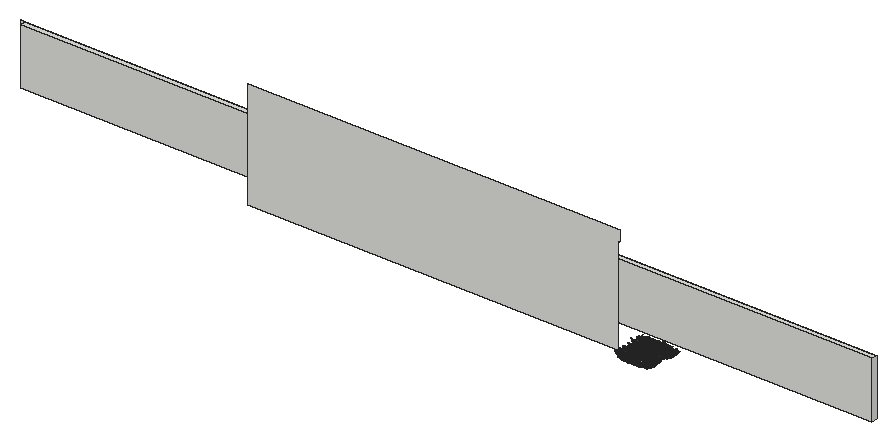
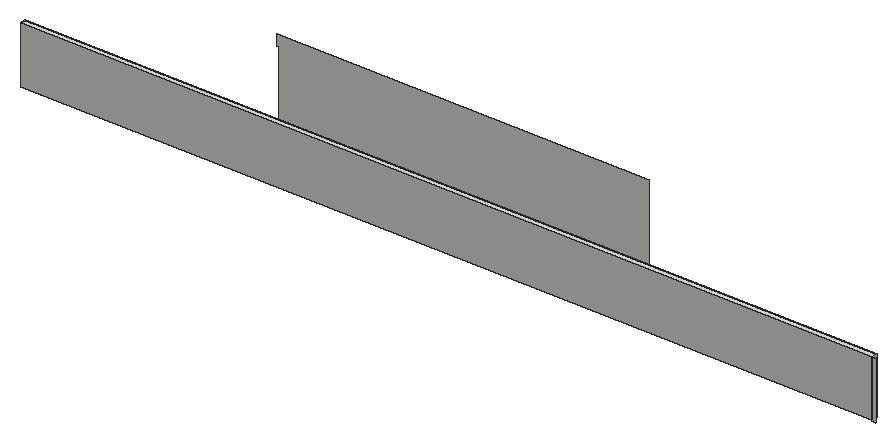
# SketchUp Ruby script. Lengths in inches.
U = 1.inch
M = Sketchup.active_model
def pt(a) = Geom::Point3d.new(a.map { |v| v * U })
def face(e, loops, mat)
  f = e.add_face(loops[0].map { |a| pt(a) })
  loops[1..].each { |l| e.add_face(l.map { |a| pt(a) }).erase! }
  f.material = f.back_material = mat if mat
  f
end
# faces: each face lists its corners as indices into pts; further lists are holes
def faces(e, pts, list, mat = nil) = list.each { |f| face(e, (f[0].is_a?(Array) ? f : [f]).map { |l| l.map { |i| pts[i] } }, mat) }
# xy, xz, yz: faces in a plane at the given z, y or x. An outline is a flat list of corners, or four numbers for a rectangle; further outlines are holes
def ring(l) = l.size == 4 ? [[l[0], l[1]], [l[2], l[1]], [l[2], l[3]], [l[0], l[3]]] : l.each_slice(2).to_a
def flat(e, list, mat, &to3) = list.each { |f| face(e, (f[0].is_a?(Array) ? f : [f]).map { |l| ring(l).map { |u, v| to3.(u, v) } }, mat) }
def xy(e, z, list, mat = nil) = flat(e, list, mat) { |x, y| [x, y, z] }
def xz(e, y, list, mat = nil) = flat(e, list, mat) { |x, z| [x, y, z] }
def yz(e, x, list, mat = nil) = flat(e, list, mat) { |y, z| [x, y, z] }
def lines(e, pts, list) = list.each { |a, b| e.add_line(pt(pts[a]), pt(pts[b])) }
# prism: a flat outline (further loops are holes) pulled along v
def prism(e, loops, v, mat = nil)
  f = face(e, loops, mat); d = Geom::Vector3d.new(v.map { |x| x * U })
  f.pushpull(f.normal.samedirection?(d) ? d.length : -d.length)
end
def box(e, o, s, mat = nil) = prism(e, [[o, [o[0] + s[0], o[1], o[2]], [o[0] + s[0], o[1] + s[1], o[2]], [o[0], o[1] + s[1], o[2]]]], [0, 0, s[2]], mat)
def at(x, y, z, deg = 0) = Geom::Transformation.translation(pt([x, y, z])) * Geom::Transformation.rotation(ORIGIN, Z_AXIS, deg.degrees)
def axes(o, x, y, z) = Geom::Transformation.new([*x, 0, *y, 0, *z, 0, *pt(o).to_a, 1])
def part(name) = M.definitions.add(name)
# library, detail: a bought-in or finely detailed component or shape, given as its bounding box
def library(name, o, s) = part(name).tap { |d| box(d.entities, o, s) }
def detail(e, o, s) = box(e.add_group.entities, o, s)
def put(e, d, t, mat = nil) = e.add_instance(d, t).tap { |i| i.material = mat if mat }
def group(e, t, mat = nil) = e.add_group.tap { |g| g.transformation = t; g.material = mat if mat }.entities
root = M.entities
M.materials.add("Material10").color = [48, 100, 38]
M.materials.add("Material3").color = [68, 110, 58]
M.materials.add("Material4").color = [48, 90, 38]
M.materials.add("Material5").color = [68, 110, 48]
M.materials.add("Material6").color = [48, 90, 48]
M.materials.add("Material7").color = [58, 110, 58]
M.materials.add("Material8").color = [58, 90, 38]
M.materials.add("Material9").color = [68, 100, 58]
c1 = part("grass00")
p = [[-0.6875,0.15,0],[-0.56,0.08,5.52],[-0.04,0.03,2.76],[0.48,-0.02,0],[0.35,-0.02,5.52],[-0.1,-0.14,5.52],
  [-0.12,0.65,8.37],[-0.42,0.65,8.37]]
faces(c1.entities,p,[[0,1,2,3],[3,2,4],[1,5,2],[5,4,2],[1,6,5],[4,5,6],[7,6,1]])
c2 = part("Group16\#1")
put(c2.entities,c1,axes([1.44,-0.61,-0.01],[0.05352,0.12609,0],[-0.10704,0.04543,0.07239],[0.06664,-0.02828,0.11628]),"Material6")
put(c2.entities,c1,axes([0.76,-0.15,-0.01],[0.04676,0.24062,0],[-0.23162,0.04501,0.06642],[0.0652,-0.01267,0.23595]),"Material3")
put(c2.entities,c1,axes([0.79,0.01,-0.01],[-0.00606,0.34651,0],[-0.34381,-0.00602,0.0432],[0.04319,0.00076,0.34386]))
put(c2.entities,c1,axes([1,0.23,-0.01],[-0.07192,0.31144,0],[-0.28722,-0.06632,0.1236],[0.12043,0.02781,0.29478]),"Material5")
put(c2.entities,c1,axes([1.66,0.77,-0.01],[-0.13828,0.29651,0],[-0.21551,-0.1005,0.22471],[0.20365,0.09498,0.23779]),"Material10")
put(c2.entities,c1,axes([0.6875,0.52,-0.01],[-0.18126,0.24051,0],[-0.22746,-0.17142,0.09788],[0.07817,0.05891,0.28481]),"Material5")
put(c2.entities,c1,axes([0.68,0.78,-0.01],[-0.215,0.18688,0],[-0.12385,-0.14248,0.21334],[0.13995,0.16101,0.18878]),"Material3")
put(c2.entities,c1,axes([0.56,1,-0.01],[-0.13756,0.07624,0],[-0.06159,-0.11112,0.0927],[0.04494,0.08108,0.12705]),"Material5")
put(c2.entities,c1,axes([0.2,0.64,-0.01],[-0.23729,0.07254,0],[-0.05711,-0.18681,0.153],[0.04473,0.14632,0.19535]),"Material10")
put(c2.entities,c1,axes([0.0625,0.72,-0.01],[-0.28874,0.02525,0],[-0.02179,-0.24916,0.14647],[0.01276,0.14591,0.25012]),"Material3")
put(c2.entities,c1,axes([-0.08,0.62,-0.01],[-0.34089,-0.04187,0],[0.03255,-0.26504,0.216],[-0.02633,0.21439,0.26703]),"Material10")
put(c2.entities,c1,axes([-0.34,0.98,-0.01],[-0.14314,-0.0493,0],[0.04397,-0.12769,0.06843],[-0.02228,0.0647,0.13505]),"Material10")
put(c2.entities,c1,axes([-0.87,1.45,-0.01],[-0.23488,-0.14114,0],[0.13761,-0.22901,0.06087],[-0.03135,0.05217,0.26717]))
put(c2.entities,c1,axes([-0.72,0.77,-0.01],[-0.14208,-0.13251,0],[0.07209,-0.0773,0.16301],[-0.11118,0.11922,0.1057]),"Material10")
put(c2.entities,c1,axes([-0.62,0.43,-0.01],[-0.14845,-0.21203,0],[0.18654,-0.13061,0.12304],[-0.10079,0.07057,0.22772]),"Material3")
put(c2.entities,c1,axes([-0.68,0.29,-0.01],[-0.13639,-0.32136,0],[0.31723,-0.13464,0.05579],[-0.05136,0.0218,0.34462]),"Material4")
put(c2.entities,c1,axes([-0.64,0.125,-0.01],[-0.0458,-0.23569,0],[0.22124,-0.043,0.08276],[-0.08124,0.01579,0.22538]),"Material7")
put(c2.entities,c1,axes([-1.6,-0.03,-0.01],[0.00576,-0.32897,0],[0.27526,0.00482,0.18018],[-0.18015,-0.00315,0.2753]),"Material5")
put(c2.entities,c1,axes([-1.36,-0.31,-0.01],[0.05718,-0.24765,0],[0.18172,0.04196,0.17267],[-0.16825,-0.03885,0.1865]),"Material10")
put(c2.entities,c1,axes([-1.54,-0.72,-0.01],[0.06537,-0.14017,0],[0.13555,0.06321,0.03939],[-0.0357,-0.01665,0.14956]))
put(c2.entities,c1,axes([-1.19,-0.9,-0.01],[0.09597,-0.12735,0],[0.11214,0.08451,0.07557],[-0.06035,-0.04548,0.14042]),"Material9")
put(c2.entities,c1,axes([-0.47,-0.54,-0.01],[0.11588,-0.10072,0],[0.0618,0.0711,0.12124],[-0.07953,-0.0915,0.0942]))
put(c2.entities,c1,axes([-0.47,-0.84,-0.01],[0.11927,-0.0661,0],[0.06603,0.11913,0.00646],[-0.00313,-0.00565,0.13621]),"Material5")
put(c2.entities,c1,axes([-0.38,-1.24,-0.01],[0.28037,-0.08571,0],[0.0618,0.20215,0.20315],[-0.05939,-0.19428,0.21139]),"Material9")
put(c2.entities,c1,axes([-0.06,-0.66,-0.01],[0.22719,-0.01987,0],[0.01247,0.14255,0.17758],[-0.01547,-0.17691,0.1431]),"Material8")
put(c2.entities,c1,axes([0.11,-0.89,-0.01],[0.14882,0.01828,0],[-0.01058,0.08611,0.12229],[0.01491,-0.12138,0.08676]),"Material6")
put(c2.entities,c1,axes([0.25,-0.72,-0.01],[0.20481,0.07053,0],[-0.06206,0.18022,0.10291],[0.03351,-0.0973,0.1906]),"Material6")
put(c2.entities,c1,axes([0.85,-1.42,-0.01],[0.16481,0.09904,0],[-0.09472,0.15762,0.05616],[0.02893,-0.04814,0.18389]),"Material5")
put(c2.entities,c1,axes([1.01,-1.09,-0.01],[0.21858,0.20385,0],[-0.17495,0.1876,0.15339],[0.10462,-0.11218,0.25652]),"Material10")
put(c2.entities,c1,axes([1.01,-0.71,-0.01],[0.08733,0.12473,0],[-0.06445,0.04512,0.13037],[0.1068,-0.07477,0.07867]),"Material6")
c3 = part("Group15\#1")
put(c3.entities,c2,at(0,0,0))
c4 = part("3darcstudiotree_grass00\#1")
put(c4.entities,c3,at(0,0,0))
box(root,[6.4375,983.47,0],[1101.25,7.5,73.43])
xz(root,939.04,[[336.5625,0,336.5625,140.0625,817.6875,140.0625,817.6875,126.33,814.625,126.33,814.625,0]])
xz(root,990.97,[[0.875,-0.51,0.75,73.42,6.1,73.43,6.22,-0.5]])
put(root,c4,axes([829.59,942.51,0],[-3.35209,-0.40812,0],[1.8256,-0.93715,-0.03924],[0.12725,-0.06532,1.93013]))
put(root,c4,axes([829.7,933.91,0],[3.10625,-0.85798,0],[3.45102,0.78089,-0.01132],[0.05281,0.01195,1.83032]))
put(root,c4,axes([830.77,957.72,0],[0.47327,-1.08686,0],[4.60722,0.12539,-0.01362],[0.07238,0.00197,1.54899]))
put(root,c4,axes([830.25,960.43,0],[-3.67097,0.66942,0],[-2.79157,-0.95678,-0.03459],[-0.12687,-0.04348,1.84283]))
put(root,c4,axes([831.375,965.12,0],[-1.67308,-0.99744,0],[3.57228,-0.3745,-0.00949],[0.05914,-0.0062,1.63563]))
put(root,c4,axes([830.22,966.68,0],[-2.74123,0.86634,0],[-3.57969,-0.70792,-0.0328],[-0.11955,-0.02364,1.32564]))
put(root,c4,axes([831.31,945.71,0],[-4.42043,-0.11266,0],[0.48566,-1.19101,-0.03002],[0.01626,-0.03988,1.59842]))
put(root,c4,axes([830.48,971.28,0],[-1.61796,0.93996,0],[-3.84011,-0.41313,-0.01574],[-0.09207,-0.00991,1.66349]))
put(root,c4,axes([830.97,949.04,0],[3.17321,-0.79133,0],[2.66412,0.66769,-0.0036],[0.01703,0.00427,1.5794]))
put(root,c4,axes([830.39,930.3,0],[-2.36821,1.01615,0],[-4.30311,-0.62679,-0.00219],[-0.01,-0.00146,1.64693]))
put(root,c4,axes([830.1,961.78,0],[3.39555,0.33213,0],[-1.83469,1.1723,-0.03882],[-0.07009,0.04479,1.55956]))
put(root,c4,axes([831.21,969.25,0],[-2.84065,0.70186,0],[-3.36417,-0.85098,-0.01852],[-0.06548,-0.01656,1.50457]))
put(root,c4,axes([830.88,936.79,0],[4.32578,-0.20958,0],[0.90693,1.16992,-0.01483],[0.01432,0.01847,1.51152]))
put(root,c4,axes([830.55,951.89,0],[3.67456,0.57849,0],[-2.21589,0.8797,-0.03908],[-0.14607,0.05799,1.82303]))
put(root,c4,axes([831.36,940.89,0],[3.12654,0.99148,0],[-3.05993,0.60307,-0.04305],[-0.21095,0.04158,1.51958]))
put(root,c4,axes([833.03,930.32,0],[0.40076,-1.15293,0],[4.50783,0.09793,-0.03115],[0.17233,0.00374,1.5702]))
put(root,c4,axes([833.63,927.24,0],[1.18754,-1.01824,0],[3.81557,0.27812,-0.01207],[0.07759,0.00566,1.66287]))
put(root,c4,axes([834.05,967,0],[-3.92204,-0.29054,0],[1.17803,-0.99389,-0.05017],[0.08482,-0.07156,1.54202]))
put(root,c4,axes([834.51,960.5625,0],[-2.30872,-1.02741,0],[3.84342,-0.53979,-0.0488],[0.20495,-0.02878,1.32723]))
put(root,c4,axes([833.21,956.45,0],[4.53918,0.22078,0],[-0.91725,1.17863,-0.03864],[-0.04554,0.05852,1.85268]))
put(root,c4,axes([833.45,934.7,0],[4.62634,0.00391,0],[-0.01264,0.9349,-0.00416],[-0.00008,0.00596,1.3392]))
put(root,c4,axes([833.41,936.45,0],[3.44705,0.83738,0],[-3.43715,0.8843,-0.06236],[-0.26248,0.06753,1.86199]))
put(root,c4,axes([835.375,971.51,0],[-2.93,-0.68293,0],[3.05684,-0.81968,-0.04642],[0.17067,-0.04577,1.51042]))
put(root,c4,axes([834.85,954.2,0],[1.34292,-0.85261,0],[4.14174,0.40772,-0.0431],[0.19924,0.01961,1.38217]))
put(root,c4,axes([833.62,928.55,0],[-0.4238,1.09775,0],[-5.15842,-0.12447,-0.01578],[-0.06645,-0.0016,1.37044]))
put(root,c4,axes([834.91,945.22,0],[2.29787,-0.71294,0],[3.86866,0.77932,-0.04335],[0.16802,0.03385,1.54559]))
put(root,c4,axes([835.59,965.41,0],[-1.22669,-1.03547,0],[3.63714,-0.2693,-0.01669],[0.12283,-0.00909,1.82011]))
put(root,c4,axes([834.77,942.76,0],[-2.98365,0.86497,0],[-3.89047,-0.83874,-0.04683],[-0.20597,-0.0444,1.86493]))
put(root,c4,axes([835.97,963.4375,0],[-4.10256,-0.1973,0],[0.74416,-0.9671,-0.01319],[0.01782,-0.02316,1.76124]))
put(root,c4,axes([834.2,946.93,0],[4.13068,0.36881,0],[-1.71772,1.2024,-0.02984],[-0.04889,0.03422,1.55474]))
put(root,c4,axes([836.04,931.98,0],[0.06879,-0.93707,0],[3.83645,0.0176,-0.01436],[0.09429,0.00043,1.57494]))
put(root,c4,axes([835.99,944.06,0],[0.7791,-0.92292,0],[4.72913,0.24951,-0.04294],[0.18667,0.00985,1.34209]))
put(root,c4,axes([836.58,967.83,0],[-4.4686,-0.23956,0],[0.88176,-1.02798,-0.03168],[0.03699,-0.04313,1.46389]))
put(root,c4,axes([836.3,948.97,0],[1.878,-0.85136,0],[4.01986,0.55421,-0.00061],[0.00361,0.0005,1.94394]))
put(root,c4,axes([836.67,950.37,0],[1.24313,-0.92825,0],[4.47227,0.37433,-0.04023],[0.17657,0.01478,1.36415]))
put(root,c4,axes([835.65,953.15,0],[-2.14811,0.98739,0],[-4.23231,-0.57547,-0.01158],[-0.04996,-0.00679,1.47884]))
put(root,c4,axes([837.1875,957.44,0],[-0.51909,-1.27053,0],[4.17352,-0.10657,-0.01024],[0.07103,-0.00181,1.82793]))
put(root,c4,axes([836.59,933.89,0],[-2.15627,0.7748,0],[-3.75013,-0.65229,-0.02835],[-0.11927,-0.02075,1.46355]))
put(root,c4,axes([835.89,959.36,0],[-0.2443,0.90017,0],[-4.80232,-0.08146,-0.00038],[-0.00184,-0.00003,1.44006]))
put(root,c4,axes([836.24,961.62,0],[3.055,0.70222,0],[-2.89109,0.7861,-0.04265],[-0.20546,0.05586,1.90027]))
put(root,c4,axes([836.56,951.51,0],[-2.4391,1.11365,0],[-4.52145,-0.61893,-0.00813],[-0.02921,-0.004,1.31962]))
put(root,c4,axes([836.9375,940.72,0],[-2.85701,0.97241,0],[-3.78392,-0.69484,-0.02364],[-0.12588,-0.02312,1.93862]))
put(root,c4,axes([837.35,939.95,0],[3.76686,-0.83119,0],[3.36509,0.95314,-0.00351],[0.01175,0.00333,1.60808]))
put(root,c4,axes([837.38,938.34,0],[2.81917,-0.76619,0],[3.32904,0.76557,-0.05921],[0.2958,0.06802,1.91907]))
put(root,c4,axes([837.39,969.78,0],[-2.30663,1.06552,0],[-4.23551,-0.57306,-0.04902],[-0.25303,-0.03424,1.76654]))
put(root,c4,axes([839.48,951.86,0],[-1.10466,-1.04309,0],[4.11781,-0.27255,-0.00114],[0.00731,-0.00048,1.77079]))
put(root,c4,axes([839.1,927.15,0],[-1.11853,-1.11565,0],[3.68055,-0.23063,-0.0349],[0.26302,-0.01648,1.84282]))
put(root,c4,axes([839.8,942.57,0],[-4.80824,-0.47237,0],[1.62347,-1.03284,-0.03326],[0.06769,-0.04306,1.54402]))
put(root,c4,axes([839.79,952.82,0],[-4.86512,0.05083,0],[-0.1686,-1.00853,-0.02048],[-0.00677,-0.04048,1.99696]))
put(root,c4,axes([839.25,949.89,0],[-3.02468,0.58391,0],[-2.63511,-0.85312,-0.02049],[-0.06609,-0.0214,1.42185]))
put(root,c4,axes([839.8,960.77,0],[2.33832,-0.89865,0],[3.29868,0.53645,-0.01966],[0.11007,0.0179,1.64285]))
put(root,c4,axes([840.01,932.3125,0],[-3.61794,0.71954,0],[-3.11711,-0.97958,-0.00639],[-0.02051,-0.00644,1.6128]))
put(root,c4,axes([840.49,966.5,0],[-3.01459,0.57554,0],[-2.90712,-0.95168,-0.0597],[-0.23401,-0.07661,1.93343]))
put(root,c4,axes([840,970.125,0],[-1.87724,0.90474,0],[-4.04075,-0.52401,-0.04385],[-0.19356,-0.0251,1.41492]))
put(root,c4,axes([840.55,961.92,0],[-2.76695,1.05816,0],[-3.42506,-0.55976,-0.05029],[-0.32743,-0.05351,1.98932]))
put(root,c4,axes([840.9,958.97,0],[1.10502,-1.02921,0],[4.51643,0.30307,-0.05256],[0.2763,0.01854,1.59089]))
put(root,c4,axes([841.44,929.9,0],[-1.47695,-1.05774,0],[4.67611,-0.40809,-0.05387],[0.24046,-0.02099,1.46363]))
put(root,c4,axes([841.38,965.16,0],[-0.89548,-0.9705,0],[4.23678,-0.24433,-0.03351],[0.19208,-0.01108,1.59864]))
put(root,c4,axes([839.9,938.02,0],[4.62222,-0.11265,0],[0.48715,1.24932,-0.00515],[0.00288,0.00739,1.80879]))
put(root,c4,axes([842.22,935.93,0],[-4.55832,-0.10477,0],[0.39974,-1.08695,-0.01686],[0.00782,-0.02126,1.38194]))
put(root,c4,axes([840.78,947.49,0],[-0.72748,0.92095,0],[-4.90606,-0.24221,-0.01512],[-0.08825,-0.00436,1.85999]))
put(root,c4,axes([842.49,941.35,0],[1.03269,-0.98427,0],[4.16593,0.27318,-0.01105],[0.06051,0.00397,1.52421]))
put(root,c4,axes([840.91,935,0],[1.02056,1.16632,0],[-3.98079,0.21771,-0.00261],[-0.01671,0.00091,1.6704]))
put(root,c4,axes([840.9,957.84,0],[2.79724,0.70196,0],[-3.39919,0.84659,-0.03194],[-0.10291,0.02563,1.36388]))
put(root,c4,axes([842.45,933.01,0],[1.85003,-0.9013,0],[4.03488,0.51763,-0.0206],[0.11343,0.01455,1.75423]))
put(root,c4,axes([843.1875,945.71,0],[-4.31262,-0.5264,0],[2.25127,-1.15275,-0.06565],[0.15274,-0.07821,1.70067]))
put(root,c4,axes([843.41,971.47,0],[-1.35682,-1.23326,0],[4.57935,-0.31489,-0.02011],[0.12844,-0.00883,1.9663]))
put(root,c4,axes([841.43,948.28,0],[-0.08255,1.17083,0],[-4.86044,-0.02142,-0.00958],[-0.04676,-0.00021,1.48335]))
put(root,c4,axes([841.84,963.15,0],[4.4348,0.59016,0],[-2.24354,1.0537,-0.02998],[-0.09351,0.04392,1.98098]))
put(root,c4,axes([842.34,939.84,0],[0.34603,1.04205,0],[-3.81852,0.07925,-0.00998],[-0.05603,0.00116,1.34846]))
put(root,c4,axes([843.24,956.56,0],[3.30812,-0.80284,0],[2.65209,0.683,-0.02978],[0.12492,0.03217,1.43312]))
put(root,c4,axes([842.64,954.1,0],[3.9282,0.38594,0],[-1.52945,0.97295,-0.02634],[-0.05842,0.03716,1.58474]))
put(root,c4,axes([843.33,943.39,0],[3.43387,-0.66059,0],[2.3393,0.76,-0.03629],[0.13053,0.04241,1.41389]))
put(root,c4,axes([842.9,928.55,0],[2.87995,0.68544,0],[-2.96423,0.77841,-0.04733],[-0.16011,0.04205,1.31836]))
put(root,c4,axes([843.47,968.45,0],[3.76187,0.14522,0],[-0.63051,1.02078,-0.03647],[-0.03383,0.05478,1.56991]))
put(root,c4,axes([845.38,955.625,0],[-4.18758,-0.22232,0],[0.96219,-1.13271,-0.02543],[0.02933,-0.03453,1.60712]))
put(root,c4,axes([846.26,951.8,0],[-1.50965,-1.02726,0],[3.51869,-0.32319,-0.02344],[0.12593,-0.01157,1.34096]))
put(root,c4,axes([846.08,972.29,0],[-4.14711,0.13047,0],[-0.48074,-0.95501,-0.01354],[-0.00996,-0.01978,1.41676]))
put(root,c4,axes([846.01,939.48,0],[-3.93065,0.22936,0],[-0.83099,-0.89006,-0.0198],[-0.02909,-0.03116,1.47686]))
put(root,c4,axes([845.83,952.99,0],[1.12797,-1.08226,0],[3.79109,0.24695,-0.04641],[0.27021,0.0176,1.47323]))
put(root,c4,axes([846.64,949.84,0],[0.07706,-1.18991,0],[5.14858,0.02084,-0.02796],[0.13847,0.00056,1.59394]))
put(root,c4,axes([846.76,948.08,0],[-4.65628,0.436,0],[-1.28176,-0.85553,-0.01358],[-0.03081,-0.02057,1.47772]))
put(root,c4,axes([847.16,947,0],[-4.55351,-0.01078,0],[0.04878,-1.28737,-0.04475],[0.00189,-0.04985,1.43393]))
put(root,c4,axes([847.2,930.24,0],[-0.42773,-1.06924,0],[4.56175,-0.11405,-0.04439],[0.21496,-0.00537,1.39437]))
put(root,c4,axes([846.44,957.91,0],[3.27668,-0.61327,0],[2.78187,0.92896,-0.01707],[0.06911,0.02308,1.96039]))
put(root,c4,axes([847.375,945.79,0],[-4.03083,-0.21133,0],[0.96222,-1.14709,-0.00999],[0.00968,-0.01153,1.38276]))
put(root,c4,axes([845.93,963.66,0],[4.2465,-0.26624,0],[0.87998,0.87721,-0.03452],[0.06922,0.06901,1.86367]))
put(root,c4,axes([846.36,929.21,0],[4.54148,-0.35569,0],[1.42907,1.14041,-0.0458],[0.08138,0.06494,1.7756]))
put(root,c4,axes([846.98,955.12,0],[-2.58663,0.93393,0],[-3.19563,-0.55317,-0.03104],[-0.18757,-0.03247,1.78553]))
put(root,c4,axes([847.5,937.92,0],[3.25384,-0.82472,0],[2.88656,0.71179,-0.00165],[0.00841,0.00207,1.81884]))
put(root,c4,axes([846.71,961.85,0],[4.50216,0.32859,0],[-1.15691,0.9907,-0.03197],[-0.04777,0.04091,1.37583]))
put(root,c4,axes([847.76,931.74,0],[3.27706,-0.90756,0],[3.76471,0.84961,-0.0538],[0.17294,0.03903,1.37259]))
put(root,c4,axes([848.77,969.81,0],[-3.56236,-0.42367,0],[2.09245,-1.09962,-0.03826],[0.09877,-0.05191,1.82966]))
put(root,c4,axes([848.63,934.82,0],[-1.82775,-1.1638,0],[4.23116,-0.41531,-0.05278],[0.32118,-0.03153,1.85719]))
put(root,c4,axes([848.76,935.875,0],[-4.77315,-0.10069,0],[0.4015,-1.18962,-0.02802],[0.01422,-0.04212,1.8014]))
put(root,c4,axes([847.33,943.68,0],[4.00974,0.00197,0],[-0.00725,0.92038,-0.0306],[-0.0005,0.06325,1.9022]))
put(root,c4,axes([849.01,927.09,0],[0.8013,-1.18093,0],[4.91736,0.20854,-0.00997],[0.04679,0.00198,1.48373]))
put(root,c4,axes([848.88,942.73,0],[-3.72919,-0.05138,0],[0.24763,-1.12327,-0.00601],[0.00211,-0.00957,1.79325]))
put(root,c4,axes([848.97,966.21,0],[1.19738,-1.09661,0],[4.52965,0.30912,-0.00598],[0.02664,0.00182,1.35627]))
put(root,c4,axes([848.18,965.69,0],[3.65568,-0.70914,0],[2.22099,0.71559,-0.00126],[0.00457,0.00147,1.3431]))
put(root,c4,axes([848.58,970.78,0],[2.61731,-0.86986,0],[3.89148,0.73181,-0.05537],[0.21942,0.04126,1.50911]))
put(root,c4,axes([848,967.97,0],[3.93859,-0.14638,0],[0.69101,1.16209,-0.00967],[0.00686,0.01153,1.41667]))
put(root,c4,axes([847.78,933.48,0],[1.45046,1.05694,0],[-4.51111,0.38692,-0.02597],[-0.16209,0.0139,1.96681]))
put(root,c4,axes([847.78,941.26,0],[3.4597,0.79761,0],[-3.28778,0.89131,-0.03053],[-0.13377,0.03626,1.95907]))
put(root,c4,axes([849,960.78,0],[-2.65201,0.65355,0],[-3.42376,-0.86832,-0.05994],[-0.20928,-0.05308,1.51606]))
put(root,c4,axes([848.09,959.26,0],[2.03961,1.07438,0],[-3.7474,0.44463,-0.01135],[-0.07143,0.00848,1.80626]))
put(root,c4,axes([851.6,959.62,0],[-4.36276,-0.41418,0],[1.61781,-1.06507,-0.04397],[0.10568,-0.06958,1.92843]))
put(root,c4,axes([851.11,936.2,0],[4.18598,-0.49036,0],[1.98476,1.05894,-0.00986],[0.01957,0.01044,1.36783]))
put(root,c4,axes([851.61,969.91,0],[2.56056,-0.98432,0],[3.11203,0.50597,-0.04791],[0.30541,0.04966,1.76421]))
put(root,c4,axes([851.86,933.43,0],[-2.25026,0.83212,0],[-3.28634,-0.55544,-0.04556],[-0.29795,-0.05036,1.95702]))
put(root,c4,axes([851.36,960.1875,0],[4.24107,-0.51199,0],[1.69937,0.8798,-0.04306],[0.14953,0.07741,1.95064]))
put(root,c4,axes([852.16,948.28,0],[-3.84253,0.80536,0],[-2.94777,-0.87903,-0.04843],[-0.1539,-0.04589,1.41858]))
put(root,c4,axes([851.49,944.4,0],[3.94053,-0.29196,0],[1.05758,0.89211,-0.03127],[0.05685,0.04795,1.48816]))
put(root,c4,axes([851.49,942.625,0],[-1.53168,1.15293,0],[-4.14234,-0.34395,-0.00679],[-0.03089,-0.00256,1.30662]))
put(root,c4,axes([852.37,951.63,0],[2.91217,-0.96079,0],[3.36935,0.63829,-0.04967],[0.26034,0.04932,1.73743]))
put(root,c4,axes([851.68,963.81,0],[3.5038,0.25818,0],[-1.36394,1.15688,-0.04213],[-0.05636,0.0478,1.42653]))
put(root,c4,axes([851.7,939.11,0],[3.5404,0.59381,0],[-2.40006,0.89434,-0.0468],[-0.15546,0.05793,1.60535]))
put(root,c4,axes([852.01,927.74,0],[1.62948,0.92472,0],[-3.84092,0.42301,-0.02705],[-0.14541,0.01601,1.54111]))
put(root,c4,axes([852.48,962.1,0],[0.13139,0.97083,0],[-4.91867,0.04161,-0.06181],[-0.35555,0.00301,1.77032]))
put(root,c4,axes([853.59,957.84,0],[0.40983,-1.2299,0],[4.04007,0.08414,-0.04948],[0.34314,0.00715,1.76318]))
put(root,c4,axes([852.92,956.14,0],[-1.3481,0.99436,0],[-4.38162,-0.37127,-0.05878],[-0.26746,-0.02266,1.38915]))
put(root,c4,axes([854.32,954.77,0],[-4.22259,-0.42472,0],[1.51539,-0.94162,-0.02256],[0.05153,-0.03202,1.55256]))
put(root,c4,axes([852.69,952.6875,0],[5.02289,-0.20794,0],[0.8428,1.27239,-0.06031],[0.06068,0.09161,1.9859]))
put(root,c4,axes([852.42,966.6875,0],[3.33218,0.8255,0],[-3.60999,0.91074,-0.05903],[-0.23844,0.06015,1.83956]))
put(root,c4,axes([853.875,929.82,0],[-3.80407,0.33391,0],[-1.34486,-0.95759,-0.01418],[-0.0336,-0.02392,1.8149]))
put(root,c4,axes([852.375,946.47,0],[2.8431,0.99871,0],[-3.14486,0.55954,-0.01154],[-0.05137,0.00914,1.31865]))
put(root,c4,axes([854.05,937.92,0],[0.55232,-1.11163,0],[4.16686,0.1294,-0.05019],[0.29048,0.00902,1.53052]))
put(root,c4,axes([853.43,970.9375,0],[-1.89808,0.89436,0],[-4.05381,-0.53771,-0.05129],[-0.21186,-0.0281,1.34106]))
put(root,c4,axes([853.49,932.08,0],[4.09786,-0.28438,0],[1.1228,1.01119,-0.05393],[0.0997,0.08979,1.81331]))
put(root,c4,axes([853.28,950.39,0],[3.55839,0.29687,0],[-1.56966,1.17589,-0.04175],[-0.06486,0.04859,1.52086]))
put(root,c4,axes([855.32,968.15,0],[-3.54234,-0.75482,0],[2.45019,-0.71866,-0.02002],[0.0717,-0.02103,1.30322]))
put(root,c4,axes([853.68,940.57,0],[4.48344,-0.16058,0],[0.51704,0.90226,-0.032],[0.03977,0.0694,1.99674]))
put(root,c4,axes([854.16,935.09,0],[1.95173,0.87312,0],[-3.39618,0.47448,-0.02391],[-0.12805,0.01789,1.49173]))
put(root,c4,axes([854.17,945.35,0],[0.71334,1.19036,0],[-4.87402,0.18255,-0.01905],[-0.09604,0.0036,1.57029]))
put(root,c4,axes([855.43,928.96,0],[3.57558,-0.28511,0],[1.52231,1.19319,-0.05774],[0.1071,0.08395,1.91123]))
put(root,c4,axes([855,965.23,0],[4.42918,0.20065,0],[-0.79517,1.09706,-0.0513],[-0.05083,0.07012,1.54883]))
put(root,c4,axes([857.34,928.9,0],[-3.4834,-0.28364,0],[1.48287,-1.13821,-0.00123],[0.00249,-0.00191,1.95221]))
put(root,c4,axes([857.76,956.35,0],[-3.33998,-0.7783,0],[3.18573,-0.85444,-0.00052],[0.00217,-0.00058,1.79691]))
put(root,c4,axes([857.76,969.95,0],[0.94379,-0.92824,0],[3.72731,0.23686,-0.00558],[0.03773,0.0024,1.6757]))
put(root,c4,axes([857.68,964.74,0],[2.03979,-0.89321,0],[3.8754,0.55313,-0.00497],[0.021,0.003,1.35772]))
put(root,c4,axes([858,967.22,0],[2.39407,-0.96093,0],[3.77709,0.58814,-0.04551],[0.23245,0.0362,1.67334]))
put(root,c4,axes([857.78,958.13,0],[2.46437,0.8072,0],[-2.94216,0.5614,-0.04536],[-0.29999,0.05724,1.92466]))
put(root,c4,axes([858.37,931.47,0],[-1.21684,0.90717,0],[-3.63046,-0.30436,-0.03292],[-0.25254,-0.02117,1.93659]))
put(root,c4,axes([858.12,971.5,0],[-1.30402,1.0923,0],[-3.59141,-0.26797,-0.00408],[-0.02313,-0.00173,1.38631]))
put(root,c4,axes([859.375,959.51,0],[-0.13657,-1.25054,0],[5.17112,-0.0353,-0.06757],[0.36478,-0.00249,1.74608]))
